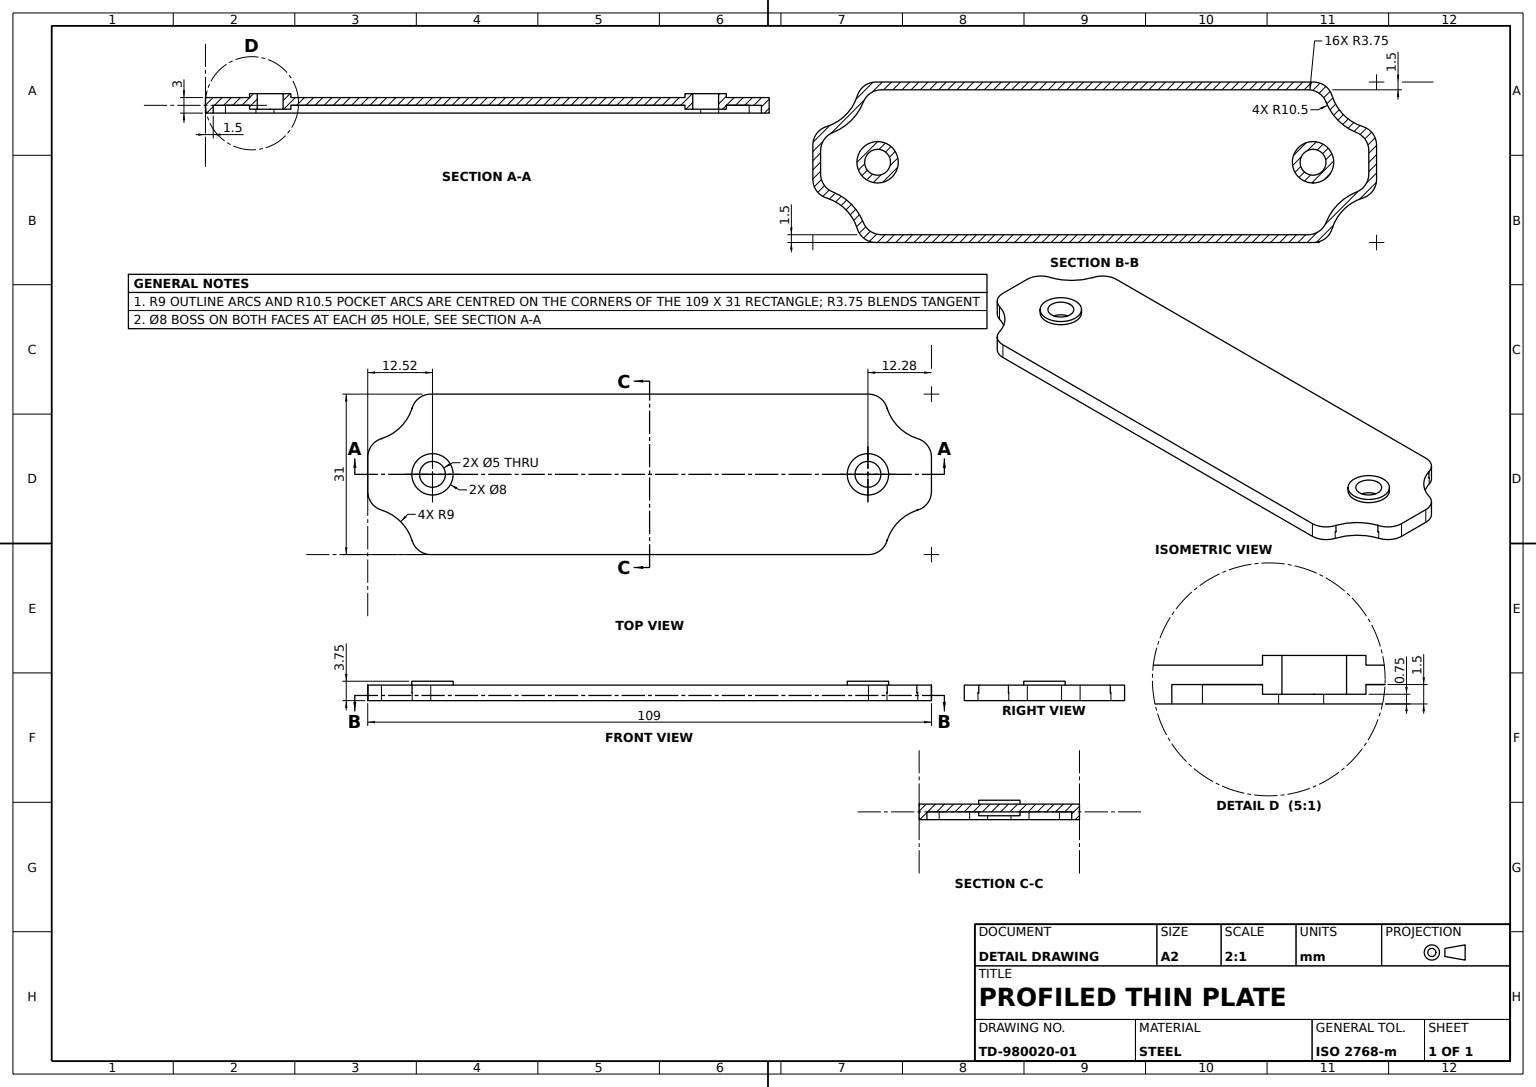
solid
v1 (45.956639,0,12.640654)
v2 (42.313942,0,15.5)
e1 v1 v2 CIRCLE(AX(P(42.313942,0,11.75),D(0,-1,0),D(0,0,1)),3.75)
v3 (42.313942,-3,15.5)
e2 v3 v2 LINE
v4 (45.898077,-3,12.852941)
e3 v3 v4 CIRCLE(AX(P(42.313942,-3,11.75),D(0,1,0),D(0,0,1)),3.75)
v5 (45.898077,-1.5,12.852941)
e4 v4 v5 LINE
v6 (45.956639,-1.5,12.640654)
e5 v5 v6 CIRCLE(AX(P(42.313942,-1.5,11.75),D(0,1,0),D(0,0,-1)),3.75)
e6 v1 v6 LINE
face CYL(AX(P(42.313942,-3,11.75),D(0,1,0),D(0,0,1)),3.75) [e1 -e2 e3 e4 e5 -e6]
v7 (-44.73858,-3,11.631579)
v8 (-41.252359,-3,14)
e7 v7 v8 CIRCLE(AX(P(-41.252359,-3,10.25),D(0,1,0),D(0,0,-1)),3.75)
v9 (-44.73858,-1.5,11.631579)
e8 v7 v9 LINE
v10 (-41.252359,-1.5,14)
e9 v9 v10 CIRCLE(AX(P(-41.252359,-1.5,10.25),D(0,1,0),D(0,0,1)),3.75)
e10 v8 v10 LINE
face CYL(AX(P(-41.252359,-3,10.25),D(0,1,0),D(0,0,1)),3.75) rev [-e7 e8 e9 -e10]
v11 (-50.631579,-3,-5.73858)
v12 (-50.631579,-1.5,-5.73858)
e11 v11 v12 LINE
v13 (-44.73858,-3,-11.631579)
e12 v13 v11 CIRCLE(AX(P(-54.5,-3,-15.5),D(0,-1,0),D(0,0,1)),10.5)
v14 (-44.73858,-1.5,-11.631579)
e13 v13 v14 LINE
e14 v14 v12 CIRCLE(AX(P(-54.5,-1.5,-15.5),D(0,-1,0),D(0,0,1)),10.5)
face CYL(AX(P(-54.5,-3,-15.5),D(0,1,0),D(0,0,1)),10.5) [-e11 -e12 e13 e14]
v15 (-51.713851,-1.5,-6.937958)
v16 (-51.852941,-1.5,-6.898077)
e15 v15 v16 CIRCLE(AX(P(-50.75,-1.5,-3.313942),D(0,1,0),D(0,0,-1)),3.75)
v17 (-51.738784,-1.5,-6.934039)
e16 v17 v15 LINE
e17 v17 v16 CIRCLE(AX(P(-54.5,-1.5,-15.5),D(0,-1,0),D(0,0,-1)),9)
face PLANE(AX(P(-50.75,-1.5,-3.313942),D(0,-1,0),D(0,0,-1))) rev [-e15 -e16 e17]
v18 (42.217054,-2.25,4)
v19 (42.217054,-2.25,-4)
e18 v18 v19 CIRCLE(AX(P(42.217054,-2.25,0),D(0,1,0),D(0,0,1)),4)
e19 v19 v18 CIRCLE(AX(P(42.217054,-2.25,0),D(0,1,0),D(0,0,1)),4)
v20 (42.217054,-2.25,-2.5)
v21 (42.217054,-2.25,2.5)
e20 v20 v21 CIRCLE(AX(P(42.217054,-2.25,0),D(0,1,0),D(0,0,1)),2.5)
e21 v21 v20 CIRCLE(AX(P(42.217054,-2.25,0),D(0,1,0),D(0,0,1)),2.5)
face PLANE(AX(P(42.217054,-2.25,0),D(0,1,0),D(0,0,1))) rev [-e18 -e19] [e20 e21]
v22 (42.217054,0,-4)
v23 (42.217054,0.75,-4)
e22 v22 v23 LINE
v24 (42.217054,0,4)
e23 v22 v24 CIRCLE(AX(P(42.217054,0,0),D(0,1,0),D(0,0,1)),4)
v25 (42.217054,0.75,4)
e24 v24 v25 LINE
e25 v23 v25 CIRCLE(AX(P(42.217054,0.75,0),D(0,1,0),D(0,0,1)),4)
face CYL(AX(P(42.217054,-2.25,0),D(0,1,0),D(0,0,1)),4) [-e22 e23 e24 -e25]
v26 (-54.5,-3,3.313942)
v27 (-54.5,0,3.313942)
e26 v26 v27 LINE
v28 (-51.852941,-3,6.898077)
e27 v26 v28 CIRCLE(AX(P(-50.75,-3,3.313942),D(0,1,0),D(0,0,-1)),3.75)
v29 (-51.852941,0,6.898077)
e28 v28 v29 LINE
e29 v29 v27 CIRCLE(AX(P(-50.75,0,3.313942),D(0,-1,0),D(0,0,1)),3.75)
face CYL(AX(P(-50.75,-3,3.313942),D(0,1,0),D(0,0,1)),3.75) [-e26 e27 e28 e29]
v30 (-41.982412,-2.25,-2.5)
v31 (-41.982412,-2.25,2.5)
e30 v30 v31 CIRCLE(AX(P(-41.982412,-2.25,0),D(0,1,0),D(0,0,1)),2.5)
e31 v31 v30 CIRCLE(AX(P(-41.982412,-2.25,0),D(0,1,0),D(0,0,1)),2.5)
v32 (-41.982412,-2.25,4)
v33 (-41.982412,-2.25,-4)
e32 v32 v33 CIRCLE(AX(P(-41.982412,-2.25,0),D(0,1,0),D(0,0,1)),4)
e33 v33 v32 CIRCLE(AX(P(-41.982412,-2.25,0),D(0,1,0),D(0,0,1)),4)
face PLANE(AX(P(-41.982412,-2.25,0),D(0,1,0),D(0,0,1))) rev [e30 e31] [-e32 -e33]
v34 (-53,-1.5,2.252359)
v35 (-50.631579,-1.5,5.73858)
e34 v34 v35 CIRCLE(AX(P(-49.25,-1.5,2.252359),D(0,1,0),D(0,0,1)),3.75)
v36 (-50.631579,-3,5.73858)
e35 v36 v35 LINE
v37 (-53,-3,2.252359)
e36 v37 v36 CIRCLE(AX(P(-49.25,-3,2.252359),D(0,1,0),D(0,0,-1)),3.75)
e37 v37 v34 LINE
face CYL(AX(P(-49.25,-3,2.252359),D(0,1,0),D(0,0,1)),3.75) rev [e34 -e35 -e36 e37]
v38 (-45.95001,-1.5,-12.667338)
v39 (-45.943102,-1.5,-12.710826)
e38 v38 v39 LINE
v40 (-45.898077,-1.5,-12.852941)
e39 v40 v38 CIRCLE(AX(P(-42.313942,-1.5,-11.75),D(0,1,0),D(0,0,-1)),3.75)
e40 v40 v39 CIRCLE(AX(P(-54.5,-1.5,-15.5),D(0,-1,0),D(0,0,-1)),9)
face PLANE(AX(P(-42.313942,-1.5,-11.75),D(0,-1,0),D(0,0,-1))) rev [-e38 -e39 e40]
e41 v35 v9 CIRCLE(AX(P(-54.5,-1.5,15.5),D(0,-1,0),D(0,0,1)),10.5)
e42 v36 v7 CIRCLE(AX(P(-54.5,-3,15.5),D(0,-1,0),D(0,0,1)),10.5)
face CYL(AX(P(-54.5,-3,15.5),D(0,1,0),D(0,0,1)),10.5) [e35 e41 -e8 -e42]
v41 (51.852941,-3,-6.898077)
v42 (45.898077,-3,-12.852941)
e43 v41 v42 CIRCLE(AX(P(54.5,-3,-15.5),D(0,-1,0),D(0,0,1)),9)
v43 (45.898077,-1.5,-12.852941)
e44 v42 v43 LINE
v44 (45.932907,-1.5,-12.742298)
e45 v44 v43 CIRCLE(AX(P(54.5,-1.5,-15.5),D(0,-1,0),D(0,0,-1)),9)
v45 (45.932907,0,-12.742298)
e46 v45 v44 LINE
v46 (51.852941,0,-6.898077)
e47 v46 v45 CIRCLE(AX(P(54.5,0,-15.5),D(0,-1,0),D(0,0,1)),9)
e48 v41 v46 LINE
face CYL(AX(P(54.5,-1.5,-15.5),D(0,1,0),D(0,0,1)),9) rev [e43 e44 -e45 -e46 -e47 -e48]
v47 (-54.5,0,-3.313942)
v48 (-51.713851,0,-6.937958)
e49 v47 v48 CIRCLE(AX(P(-50.75,0,-3.313942),D(0,-1,0),D(0,0,1)),3.75)
e50 v48 v15 LINE
v49 (-51.852941,-3,-6.898077)
e51 v49 v16 LINE
v50 (-54.5,-3,-3.313942)
e52 v49 v50 CIRCLE(AX(P(-50.75,-3,-3.313942),D(0,1,0),D(0,0,-1)),3.75)
e53 v50 v47 LINE
face CYL(AX(P(-50.75,-3,-3.313942),D(0,1,0),D(0,0,1)),3.75) [e49 e50 e15 -e51 e52 e53]
v51 (-41.982412,0.75,-2.5)
e54 v30 v51 LINE
v52 (-41.982412,0.75,2.5)
e55 v51 v52 CIRCLE(AX(P(-41.982412,0.75,0),D(0,1,0),D(0,0,1)),2.5)
e56 v31 v52 LINE
face CYL(AX(P(-41.982412,-1.5,0),D(0,1,0),D(0,0,1)),2.5) rev [-e30 e54 e55 -e56]
v53 (45.947659,-1.5,12.696885)
e57 v5 v53 CIRCLE(AX(P(54.5,-1.5,15.5),D(0,-1,0),D(0,0,-1)),9)
e58 v6 v53 LINE
face PLANE(AX(P(42.313942,-1.5,11.75),D(0,-1,0),D(0,0,-1))) rev [-e5 e57 -e58]
v54 (41.252359,-3,14)
v55 (41.252359,-1.5,14)
e59 v54 v55 LINE
e60 v8 v54 LINE
e61 v10 v55 LINE
face PLANE(AX(P(-41.252359,-3,14),D(0,0,1),D(1,0,0))) rev [-e59 -e60 e10 e61]
e62 v47 v27 LINE
e63 v50 v26 LINE
face PLANE(AX(P(-54.5,-1.5,6.5),D(-1,0,0),D(0,0,1))) [-e62 -e53 e63 e26]
v56 (53,-3,2.252359)
v57 (53,-1.5,2.252359)
e64 v56 v57 LINE
v58 (53,-1.5,-2.252359)
e65 v57 v58 LINE
v59 (53,-3,-2.252359)
e66 v59 v58 LINE
e67 v56 v59 LINE
face PLANE(AX(P(53,-3,2.252359),D(1,0,0),D(0,0,-1))) rev [e64 e65 -e66 -e67]
v60 (-41.982412,0.75,-4)
v61 (-41.982412,0.75,4)
e68 v60 v61 CIRCLE(AX(P(-41.982412,0.75,0),D(0,1,0),D(0,0,1)),4)
v62 (-41.982412,0,-4)
e69 v62 v60 LINE
v63 (-41.982412,0,4)
e70 v62 v63 CIRCLE(AX(P(-41.982412,0,0),D(0,1,0),D(0,0,1)),4)
e71 v63 v61 LINE
face CYL(AX(P(-41.982412,-2.25,0),D(0,1,0),D(0,0,1)),4) [-e68 -e69 e70 e71]
v64 (51.852941,-3,6.898077)
e72 v4 v64 CIRCLE(AX(P(54.5,-3,15.5),D(0,-1,0),D(0,0,1)),9)
v65 (51.852941,-1.5,6.898077)
e73 v64 v65 LINE
v66 (51.673566,-1.5,6.955337)
e74 v66 v65 CIRCLE(AX(P(54.5,-1.5,15.5),D(0,-1,0),D(0,0,-1)),9)
v67 (51.673566,0,6.955337)
e75 v67 v66 LINE
v68 (45.947659,0,12.696885)
e76 v68 v67 CIRCLE(AX(P(54.5,0,15.5),D(0,-1,0),D(0,0,1)),9)
e77 v53 v68 LINE
face CYL(AX(P(54.5,-1.5,15.5),D(0,1,0),D(0,0,1)),9) rev [e72 e73 -e74 -e75 -e76 -e77 -e57 -e4]
v69 (54.5,0,-3.313942)
e78 v46 v69 CIRCLE(AX(P(50.75,0,-3.313942),D(0,-1,0),D(0,0,1)),3.75)
v70 (54.5,-3,-3.313942)
e79 v70 v69 LINE
e80 v70 v41 CIRCLE(AX(P(50.75,-3,-3.313942),D(0,1,0),D(0,0,1)),3.75)
face CYL(AX(P(50.75,-3,-3.313942),D(0,1,0),D(0,0,1)),3.75) [e48 e78 -e79 e80]
v71 (-42.313942,-3,15.5)
v72 (-42.313942,0,15.5)
e81 v71 v72 LINE
e82 v71 v3 LINE
e83 v72 v2 LINE
face PLANE(AX(P(-45.5,-1.5,15.5),D(0,0,1),D(1,0,0))) [-e81 e82 e2 -e83]
e84 v68 v1 LINE
face PLANE(AX(P(45.5,1.5,15.5),D(0.987486749,0,0.157701998),D(0.157701998,0,-0.987486749))) rev [e58 e77 e84 e6]
v73 (45.936536,-1.5,-12.719185)
e85 v73 v43 CIRCLE(AX(P(42.313942,-1.5,-11.75),D(0,1,0),D(0,0,-1)),3.75)
e86 v44 v73 LINE
face PLANE(AX(P(42.313942,-1.5,-11.75),D(0,-1,0),D(0,0,-1))) rev [e45 -e85 -e86]
v74 (-41.252359,-3,-14)
e87 v74 v13 CIRCLE(AX(P(-41.252359,-3,-10.25),D(0,1,0),D(0,0,-1)),3.75)
v75 (-41.252359,-1.5,-14)
e88 v74 v75 LINE
e89 v75 v14 CIRCLE(AX(P(-41.252359,-1.5,-10.25),D(0,1,0),D(0,0,1)),3.75)
face CYL(AX(P(-41.252359,-3,-10.25),D(0,1,0),D(0,0,1)),3.75) rev [-e87 e88 e89 -e13]
v76 (51.587845,-1.5,6.969146)
e90 v66 v76 LINE
e91 v76 v65 CIRCLE(AX(P(50.75,-1.5,3.313942),D(0,1,0),D(0,0,-1)),3.75)
face PLANE(AX(P(50.75,-1.5,3.313942),D(0,-1,0),D(0,0,-1))) rev [-e90 e74 -e91]
v77 (54.5,-3,3.313942)
e92 v77 v70 LINE
e93 v64 v77 CIRCLE(AX(P(50.75,-3,3.313942),D(0,1,0),D(0,0,-1)),3.75)
v78 (-45.898077,-3,12.852941)
e94 v78 v71 CIRCLE(AX(P(-42.313942,-3,11.75),D(0,1,0),D(0,0,-1)),3.75)
e95 v28 v78 CIRCLE(AX(P(-54.5,-3,15.5),D(0,-1,0),D(0,0,1)),9)
v79 (-45.898077,-3,-12.852941)
e96 v79 v49 CIRCLE(AX(P(-54.5,-3,-15.5),D(0,-1,0),D(0,0,1)),9)
v80 (-42.313942,-3,-15.5)
e97 v80 v79 CIRCLE(AX(P(-42.313942,-3,-11.75),D(0,1,0),D(0,0,-1)),3.75)
v81 (42.313942,-3,-15.5)
e98 v81 v80 LINE
e99 v42 v81 CIRCLE(AX(P(42.313942,-3,-11.75),D(0,1,0),D(0,0,1)),3.75)
v82 (41.252359,-3,-14)
e100 v82 v74 LINE
v83 (-53,-3,-2.252359)
e101 v11 v83 CIRCLE(AX(P(-49.25,-3,-2.252359),D(0,1,0),D(0,0,-1)),3.75)
e102 v83 v37 LINE
v84 (44.73858,-3,11.631579)
e103 v54 v84 CIRCLE(AX(P(41.252359,-3,10.25),D(0,1,0),D(0,0,1)),3.75)
v85 (50.631579,-3,5.73858)
e104 v84 v85 CIRCLE(AX(P(54.5,-3,15.5),D(0,-1,0),D(0,0,1)),10.5)
e105 v85 v56 CIRCLE(AX(P(49.25,-3,2.252359),D(0,1,0),D(0,0,1)),3.75)
v86 (50.631579,-3,-5.73858)
e106 v59 v86 CIRCLE(AX(P(49.25,-3,-2.252359),D(0,1,0),D(0,0,1)),3.75)
v87 (44.73858,-3,-11.631579)
e107 v86 v87 CIRCLE(AX(P(54.5,-3,-15.5),D(0,-1,0),D(0,0,1)),10.5)
e108 v87 v82 CIRCLE(AX(P(41.252359,-3,-10.25),D(0,1,0),D(0,0,1)),3.75)
face PLANE(AX(P(42.313942,-3,-11.75),D(0,1,0),D(0,0,1))) rev [-e92 -e93 -e72 -e3 -e82 -e94 -e95 -e27 -e63 -e52 -e96 -e97 -e98 -e99 -e43 -e80] [e100 e87 e12 e101 e102 e36 e42 e7 e60 e103 e104 e105 e67 e106 e107 e108]
v88 (42.217054,-1.5,-4)
v89 (42.217054,-1.5,4)
e109 v88 v89 CIRCLE(AX(P(42.217054,-1.5,0),D(0,1,0),D(0,0,1)),4)
e110 v19 v88 LINE
e111 v18 v89 LINE
face CYL(AX(P(42.217054,-2.25,0),D(0,1,0),D(0,0,1)),4) [-e109 -e110 e19 e111]
v90 (-45.95001,0,-12.667338)
e112 v90 v38 LINE
v91 (-42.313942,0,-15.5)
e113 v90 v91 CIRCLE(AX(P(-42.313942,0,-11.75),D(0,-1,0),D(0,0,1)),3.75)
e114 v80 v91 LINE
e115 v79 v40 LINE
face CYL(AX(P(-42.313942,-3,-11.75),D(0,1,0),D(0,0,1)),3.75) [e39 -e112 e113 -e114 e97 e115]
v92 (51.587845,0,6.969146)
e116 v92 v76 LINE
e117 v92 v67 LINE
face PLANE(AX(P(54.5,1.5,6.5),D(0.159048682,0,0.987270741),D(0.987270741,0,-0.159048682))) rev [e90 -e116 e117 e75]
v93 (44.73858,-1.5,11.631579)
e118 v55 v93 CIRCLE(AX(P(41.252359,-1.5,10.25),D(0,1,0),D(0,0,1)),3.75)
e119 v84 v93 LINE
face CYL(AX(P(41.252359,-3,10.25),D(0,1,0),D(0,0,1)),3.75) rev [e118 -e119 -e103 e59]
e120 v52 v51 CIRCLE(AX(P(-41.982412,0.75,0),D(0,1,0),D(0,0,1)),2.5)
e121 v61 v60 CIRCLE(AX(P(-41.982412,0.75,0),D(0,1,0),D(0,0,1)),4)
face PLANE(AX(P(-41.982412,0.75,0),D(0,1,0),D(0,0,1))) [-e55 -e120] [e68 e121]
e122 v25 v23 CIRCLE(AX(P(42.217054,0.75,0),D(0,1,0),D(0,0,1)),4)
e123 v24 v22 CIRCLE(AX(P(42.217054,0,0),D(0,1,0),D(0,0,1)),4)
face CYL(AX(P(42.217054,-2.25,0),D(0,1,0),D(0,0,1)),4) [-e122 -e24 e123 e22]
v94 (41.252359,-1.5,-14)
e124 v82 v94 LINE
e125 v94 v75 LINE
face PLANE(AX(P(41.252359,-3,-14),D(0,0,-1),D(-1,0,0))) rev [e124 e125 -e88 -e100]
v95 (-45.943102,0,-12.710826)
e126 v95 v90 LINE
e127 v39 v95 LINE
face PLANE(AX(P(-45.5,1.5,-15.5),D(-0.987614922,0,-0.156897308),D(-0.156897308,0,0.987614922))) rev [e126 e112 e38 e127]
v96 (-45.925159,-1.5,12.76075)
v97 (-45.898077,-1.5,12.852941)
e128 v96 v97 CIRCLE(AX(P(-42.313942,-1.5,11.75),D(0,1,0),D(0,0,-1)),3.75)
e129 v78 v97 LINE
v98 (-45.925159,0,12.76075)
e130 v72 v98 CIRCLE(AX(P(-42.313942,0,11.75),D(0,-1,0),D(0,0,1)),3.75)
e131 v98 v96 LINE
face CYL(AX(P(-42.313942,-3,11.75),D(0,1,0),D(0,0,1)),3.75) [e128 -e129 e94 e81 e130 e131]
v99 (54.5,0,3.313942)
e132 v99 v69 LINE
e133 v77 v99 LINE
face PLANE(AX(P(54.5,-1.5,6.5),D(1,0,0),D(0,0,-1))) [e79 -e132 -e133 e92]
v100 (-51.738784,0,-6.934039)
e134 v100 v17 LINE
e135 v95 v100 CIRCLE(AX(P(-54.5,0,-15.5),D(0,-1,0),D(0,0,1)),9)
face CYL(AX(P(-54.5,-1.5,-15.5),D(0,1,0),D(0,0,1)),9) rev [-e17 -e134 -e135 -e127 -e40 -e115 e96 e51]
v101 (-53,-1.5,-2.252359)
e136 v101 v34 LINE
e137 v83 v101 LINE
face PLANE(AX(P(-53,-3,-2.252359),D(-1,0,0),D(0,0,1))) rev [e136 -e37 -e102 e137]
v102 (-45.923422,0,12.77194)
v103 (-45.923422,-1.5,12.77194)
e138 v102 v103 LINE
e139 v103 v96 LINE
e140 v98 v102 LINE
face PLANE(AX(P(-45.5,1.5,15.5),D(-0.988168281,0,0.153373558),D(0.153373558,0,0.988168281))) rev [e138 e139 -e131 e140]
v104 (50.631579,-1.5,5.73858)
e141 v104 v57 CIRCLE(AX(P(49.25,-1.5,2.252359),D(0,1,0),D(0,0,1)),3.75)
e142 v85 v104 LINE
face CYL(AX(P(49.25,-3,2.252359),D(0,1,0),D(0,0,1)),3.75) rev [e141 -e64 -e105 e142]
e143 v63 v62 CIRCLE(AX(P(-41.982412,0,0),D(0,1,0),D(0,0,1)),4)
e144 v48 v100 LINE
e145 v29 v102 CIRCLE(AX(P(-54.5,0,15.5),D(0,-1,0),D(0,0,1)),9)
e146 v99 v92 CIRCLE(AX(P(50.75,0,3.313942),D(0,-1,0),D(0,0,1)),3.75)
v105 (45.936536,0,-12.719185)
e147 v105 v45 LINE
v106 (42.313942,0,-15.5)
e148 v106 v105 CIRCLE(AX(P(42.313942,0,-11.75),D(0,-1,0),D(0,0,1)),3.75)
e149 v106 v91 LINE
face PLANE(AX(P(54.5,0,-15.5),D(0,1,0),D(0,0,1))) [-e70 -e143] [-e113 -e126 e135 -e144 -e49 e62 -e29 e145 -e140 -e130 e83 -e1 -e84 e76 -e117 -e146 e132 -e78 e47 -e147 -e148 e149] [-e123 -e23]
v107 (42.217054,0.75,-2.5)
v108 (42.217054,0.75,2.5)
e150 v107 v108 CIRCLE(AX(P(42.217054,0.75,0),D(0,1,0),D(0,0,1)),2.5)
e151 v108 v107 CIRCLE(AX(P(42.217054,0.75,0),D(0,1,0),D(0,0,1)),2.5)
face PLANE(AX(P(42.217054,0.75,0),D(0,1,0),D(0,0,1))) [-e150 -e151] [e25 e122]
e152 v103 v97 CIRCLE(AX(P(-54.5,-1.5,15.5),D(0,-1,0),D(0,0,-1)),9)
face PLANE(AX(P(-42.313942,-1.5,11.75),D(0,-1,0),D(0,0,-1))) rev [e152 -e128 -e139]
e153 v93 v104 CIRCLE(AX(P(54.5,-1.5,15.5),D(0,-1,0),D(0,0,1)),10.5)
face CYL(AX(P(54.5,-3,15.5),D(0,1,0),D(0,0,1)),10.5) [e119 e153 -e142 -e104]
e154 v105 v73 LINE
face PLANE(AX(P(45.5,1.5,-15.5),D(0.987901615,0,-0.155081913),D(-0.155081913,0,-0.987901615))) rev [e147 e46 e86 -e154]
face CYL(AX(P(-41.982412,-1.5,0),D(0,1,0),D(0,0,1)),2.5) rev [-e31 e56 e120 -e54]
e155 v89 v88 CIRCLE(AX(P(42.217054,-1.5,0),D(0,1,0),D(0,0,1)),4)
face CYL(AX(P(42.217054,-2.25,0),D(0,1,0),D(0,0,1)),4) [-e155 -e111 e18 e110]
face PLANE(AX(P(-54.5,1.5,-6.5),D(-0.155284513,0,-0.987869789),D(-0.987869789,0,0.155284513))) rev [-e50 e144 e134 e16]
v109 (-41.982412,-1.5,4)
v110 (-41.982412,-1.5,-4)
e156 v109 v110 CIRCLE(AX(P(-41.982412,-1.5,0),D(0,1,0),D(0,0,1)),4)
e157 v110 v109 CIRCLE(AX(P(-41.982412,-1.5,0),D(0,1,0),D(0,0,1)),4)
e158 v12 v101 CIRCLE(AX(P(-49.25,-1.5,-2.252359),D(0,1,0),D(0,0,1)),3.75)
v111 (44.73858,-1.5,-11.631579)
e159 v111 v94 CIRCLE(AX(P(41.252359,-1.5,-10.25),D(0,1,0),D(0,0,1)),3.75)
v112 (50.631579,-1.5,-5.73858)
e160 v112 v111 CIRCLE(AX(P(54.5,-1.5,-15.5),D(0,-1,0),D(0,0,1)),10.5)
e161 v58 v112 CIRCLE(AX(P(49.25,-1.5,-2.252359),D(0,1,0),D(0,0,1)),3.75)
face PLANE(AX(P(54.5,-1.5,-15.5),D(0,1,0),D(0,0,1))) rev [e156 e157] [-e158 -e14 -e89 -e125 -e159 -e160 -e161 -e65 -e141 -e153 -e118 -e61 -e9 -e41 -e34 -e136] [e155 e109]
e162 v33 v110 LINE
e163 v32 v109 LINE
face CYL(AX(P(-41.982412,-2.25,0),D(0,1,0),D(0,0,1)),4) [e32 e162 -e156 -e163]
face CYL(AX(P(-41.982412,-2.25,0),D(0,1,0),D(0,0,1)),4) [-e162 e33 e163 -e157]
face CYL(AX(P(-49.25,-3,-2.252359),D(0,1,0),D(0,0,1)),3.75) rev [e158 -e137 -e101 e11]
face CYL(AX(P(50.75,-3,3.313942),D(0,1,0),D(0,0,1)),3.75) [-e73 e93 e133 e146 e116 e91]
e164 v87 v111 LINE
e165 v86 v112 LINE
face CYL(AX(P(54.5,-3,-15.5),D(0,1,0),D(0,0,1)),10.5) [-e164 -e107 e165 e160]
face CYL(AX(P(49.25,-3,-2.252359),D(0,1,0),D(0,0,1)),3.75) rev [e161 -e165 -e106 e66]
face CYL(AX(P(-54.5,-1.5,15.5),D(0,1,0),D(0,0,1)),9) rev [-e28 e95 e129 -e152 -e138 -e145]
e166 v81 v106 LINE
face PLANE(AX(P(-45.5,-1.5,-15.5),D(0,0,-1),D(-1,0,0))) [e114 -e149 -e166 e98]
face CYL(AX(P(41.252359,-3,-10.25),D(0,1,0),D(0,0,1)),3.75) rev [-e124 -e108 e164 e159]
e167 v21 v108 LINE
e168 v20 v107 LINE
face CYL(AX(P(42.217054,-1.5,0),D(0,1,0),D(0,0,1)),2.5) rev [-e21 e167 e151 -e168]
face CYL(AX(P(42.217054,-1.5,0),D(0,1,0),D(0,0,1)),2.5) rev [-e167 -e20 e168 e150]
face CYL(AX(P(-41.982412,-2.25,0),D(0,1,0),D(0,0,1)),4) [-e71 e143 e69 -e121]
face CYL(AX(P(42.313942,-3,-11.75),D(0,1,0),D(0,0,1)),3.75) [e85 -e44 e99 e166 e148 e154]
